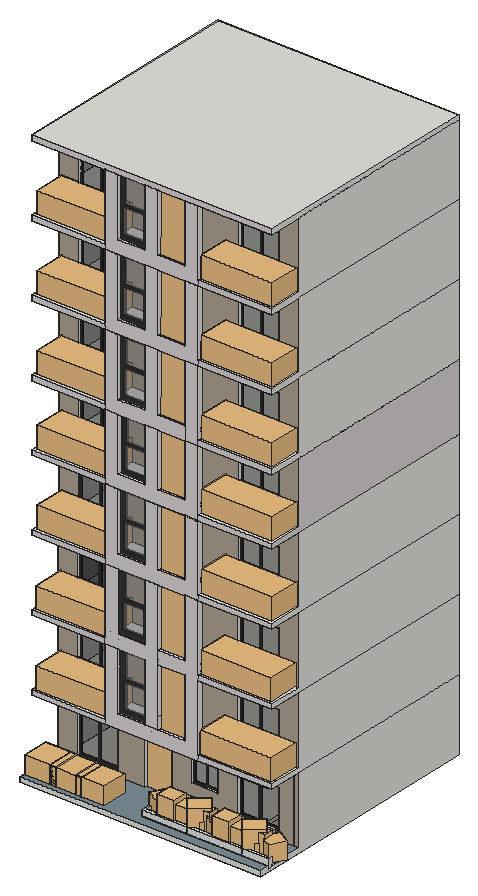
# SketchUp Ruby script. Lengths in inches.
U = 1.inch
M = Sketchup.active_model
def pt(a) = Geom::Point3d.new(a.map { |v| v * U })
def face(e, loops, mat)
  f = e.add_face(loops[0].map { |a| pt(a) })
  loops[1..].each { |l| e.add_face(l.map { |a| pt(a) }).erase! }
  f.material = f.back_material = mat if mat
  f
end
# faces: each face lists its corners as indices into pts; further lists are holes
def faces(e, pts, list, mat = nil) = list.each { |f| face(e, (f[0].is_a?(Array) ? f : [f]).map { |l| l.map { |i| pts[i] } }, mat) }
# xy, xz, yz: faces in a plane at the given z, y or x. An outline is a flat list of corners, or four numbers for a rectangle; further outlines are holes
def ring(l) = l.size == 4 ? [[l[0], l[1]], [l[2], l[1]], [l[2], l[3]], [l[0], l[3]]] : l.each_slice(2).to_a
def flat(e, list, mat, &to3) = list.each { |f| face(e, (f[0].is_a?(Array) ? f : [f]).map { |l| ring(l).map { |u, v| to3.(u, v) } }, mat) }
def xy(e, z, list, mat = nil) = flat(e, list, mat) { |x, y| [x, y, z] }
def xz(e, y, list, mat = nil) = flat(e, list, mat) { |x, z| [x, y, z] }
def yz(e, x, list, mat = nil) = flat(e, list, mat) { |y, z| [x, y, z] }
def lines(e, pts, list) = list.each { |a, b| e.add_line(pt(pts[a]), pt(pts[b])) }
# prism: a flat outline (further loops are holes) pulled along v
def prism(e, loops, v, mat = nil)
  f = face(e, loops, mat); d = Geom::Vector3d.new(v.map { |x| x * U })
  f.pushpull(f.normal.samedirection?(d) ? d.length : -d.length)
end
def box(e, o, s, mat = nil) = prism(e, [[o, [o[0] + s[0], o[1], o[2]], [o[0] + s[0], o[1] + s[1], o[2]], [o[0], o[1] + s[1], o[2]]]], [0, 0, s[2]], mat)
def at(x, y, z, deg = 0) = Geom::Transformation.translation(pt([x, y, z])) * Geom::Transformation.rotation(ORIGIN, Z_AXIS, deg.degrees)
def axes(o, x, y, z) = Geom::Transformation.new([*x, 0, *y, 0, *z, 0, *pt(o).to_a, 1])
def part(name) = M.definitions.add(name)
# library, detail: a bought-in or finely detailed component or shape, given as its bounding box
def library(name, o, s) = part(name).tap { |d| box(d.entities, o, s) }
def detail(e, o, s) = box(e.add_group.entities, o, s)
def put(e, d, t, mat = nil) = e.add_instance(d, t).tap { |i| i.material = mat if mat }
def group(e, t, mat = nil) = e.add_group.tap { |g| g.transformation = t; g.material = mat if mat }.entities
root = M.entities
M.materials.add("Glass_Tinted_Gray").color = [0, 0, 0]
M.materials["Glass_Tinted_Gray"].alpha = 0.125
M.materials.add("Material__1").color = [95, 70, 46]
M.materials.add("Windows").color = [58, 58, 58]
M.materials.add("[0035_Tan]").color = [174, 162, 146]
M.materials.add("[0135_DarkGray]").color = [81, 81, 81]
M.materials.add("[Blinds Cellular White]").color = [217, 211, 213]
M.materials.add("[Mirror 02]").color = [229, 229, 229]
M.materials.add("[Square Glass Tile 01]").color = [123, 142, 151]
M.materials.add("[Terrazzo Light Blue]").color = [196, 214, 227]
M.materials.add("[Translucent Glass Gray]").color = [128, 128, 128]
M.materials["[Translucent Glass Gray]"].alpha = 0.5
c1 = part("PENTEK_RP Fineline 50S_Sliding_DoorCase_E1")
box(c1.entities,[0,0,0],[1.51,3.66,99.27],"[0135_DarkGray]")
c2 = part("PENTEK_RP Fineline 50S_SlidingDooe_Case_E2")
box(c2.entities,[0,0,0],[96.25,3.66,1.51],"[0135_DarkGray]")
c3 = part("pentek_RP Fineline 50S_SlidingDoor_Case")
put(c3.entities,c1,at(97.76,0,0))
put(c3.entities,c2,at(1.51,0,0))
put(c3.entities,c1,at(0,0,0))
put(c3.entities,c2,at(1.51,0,97.76))
c4 = part("PENTEK_RP Fineline 50S_SlidingDoor_GlazingBead_2")
box(c4.entities,[0,0,0],[0.56,0.59,94.39],"[0135_DarkGray]")
c5 = part("PENTEK_RP Fineline 50S_SlidingDoor_Glass")
box(c5.entities,[0,0,0],[46.58,0.16,94.39],"Glass_Tinted_Gray")
c6 = part("PENTEK_RP Fineline 50S_SlidingDoor_GlazingBead")
box(c6.entities,[0,0,0],[45.47,0.59,0.56],"[0135_DarkGray]")
c7 = part("PENTEK_RP Fineline 50S_SlidingDoor_Leaf_E1")
xy(c7.entities,0,[[0,0,0.93,1.97],[0.93,1.57,1.49,1.97]],"[0135_DarkGray]")
xy(c7.entities,96.25,[[0,0,0.93,0,0.93,1.57,1.49,1.57,1.49,1.97,0,1.97]],"[0135_DarkGray]")
xz(c7.entities,0,[[0,0,0.93,96.25]],"[0135_DarkGray]")
xz(c7.entities,1.57,[[0.93,0,1.49,95.32],[0.93,95.32,1.49,96.25]],"[0135_DarkGray]")
xz(c7.entities,1.97,[[0,0,1.49,96.25]],"[0135_DarkGray]")
yz(c7.entities,0,[[0,0,1.97,96.25]],"[0135_DarkGray]")
yz(c7.entities,0.93,[[0,0,1.57,0.93],[0,0.93,1.57,95.32],[0,95.32,1.57,96.25]],"[0135_DarkGray]")
yz(c7.entities,1.49,[[1.57,0,1.97,95.32],[1.57,95.32,1.97,96.25]],"[0135_DarkGray]")
c8 = part("PENTEK_RP Fineline 50S_SlidingDoor_Leaf_E2")
xy(c8.entities,0,[[0,0,0,1.57,0.56,1.57,0.56,1.97,46.02,1.97,46.02,1.57,46.58,1.57,46.58,0]],"[0135_DarkGray]")
xy(c8.entities,0.93,[[0,0,46.58,1.57]],"[0135_DarkGray]")
xy(c8.entities,1.49,[[0.56,1.57,46.02,1.97]],"[0135_DarkGray]")
xz(c8.entities,0,[[0,0,46.58,0.93]],"[0135_DarkGray]")
xz(c8.entities,1.57,[[0,0,0.56,0.93],[46.02,0,46.58,0.93],[0.56,0.93,46.02,1.49]],"[0135_DarkGray]")
xz(c8.entities,1.97,[[0.56,0,46.02,1.49]],"[0135_DarkGray]")
yz(c8.entities,0,[[0,0,1.57,0.93]],"[0135_DarkGray]")
yz(c8.entities,0.56,[[1.57,0,1.97,0.93],[1.57,0.93,1.97,1.49]],"[0135_DarkGray]")
yz(c8.entities,46.02,[[1.57,0,1.97,0.93],[1.57,0.93,1.97,1.49]],"[0135_DarkGray]")
yz(c8.entities,46.58,[[0,0,1.57,0.93]],"[0135_DarkGray]")
c9 = part("PENTEK_RP Fineline S_SlidingDoor_Leaf1")
put(c9.entities,c4,at(0.93,0,0.93))
put(c9.entities,c4,at(46.96,0,0.93))
put(c9.entities,c5,at(1.49,1.42,0.93))
put(c9.entities,c6,at(1.49,0,0.93))
put(c9.entities,c5,at(1.49,0.59,0.93),"[Terrazzo Light Blue]")
put(c9.entities,c7,at(0,0,0))
put(c9.entities,c7,axes([48.44,0,0],[-1,0,0],[0,1,0],[0,0,1]))
put(c9.entities,c8,axes([0.93,0,96.25],[1,0,0],[0,1,0],[0,0,-1]))
put(c9.entities,c8,at(0.93,0,0))
put(c9.entities,c6,at(1.49,0,94.77))
c10 = part("PENTEK_RP Fineline 50S_SlidingDoor_Leaf2")
put(c10.entities,c5,at(1.49,1.42,0.93))
put(c10.entities,c6,at(1.49,0,94.77))
put(c10.entities,c4,at(46.96,0,0.93))
put(c10.entities,c5,at(1.49,0.59,0.93),"[Mirror 02]")
put(c10.entities,c4,at(0.93,0,0.93))
put(c10.entities,c7,at(0,0,0))
put(c10.entities,c7,axes([48.44,0,0],[-1,0,0],[0,1,0],[0,0,1]))
put(c10.entities,c6,at(1.49,0,0.93))
put(c10.entities,c8,axes([0.93,0,96.25],[1,0,0],[0,1,0],[0,0,-1]))
put(c10.entities,c8,at(0.93,0,0))
c11 = part("PENTEK - Slimmest Steel Sliding Door / Window\#1")
put(c11.entities,c3,at(0,-1.88,-0.09))
put(c11.entities,c9,at(1.51,-2.27,1.42))
put(c11.entities,c10,at(49.32,-0.3,1.42))
c12 = library("PINTU 6 YA",[0,-0.6875,0],[35.83,8.07,80.71])
c13 = library("Double casement window",[0,0,0],[5.2,55.12,70.87])
c14 = part("Window 06")
g1 = group(c14.entities,at(-11,5.5,0,-90))
xy(g1,0,[[0,11,5.5,35]],"Windows")
xy(g1,2,[[0,13,5.5,33]],"Windows")
xy(g1,53,[[0,13,5.5,33]],"Windows")
xy(g1,55,[[0,11,5.5,35]],"Windows")
xz(g1,11,[[0,0,5.5,55]],"Windows")
xz(g1,13,[[0,2,5.5,53]],"Windows")
xz(g1,33,[[0,2,5.5,53]],"Windows")
xz(g1,35,[[0,0,5.5,55]],"Windows")
yz(g1,0,[[[11,0,35,55],[13,2,33,53]]],"Windows")
yz(g1,5.5,[[[11,0,35,55],[13,2,33,53]]],"Windows")
g2 = group(g1,at(2.75,2,2))
xy(g2,0,[[0,11,2,31]],"Windows")
xy(g2,1,[[0,12,1,30],[1,12,2,30]],"Windows")
xy(g2,25,[[0,12,1,30],[1,12,2,30]],"Windows")
xy(g2,26,[[0,11,2,31]],"Windows")
xz(g2,11,[[0,0,2,26]],"Windows")
xz(g2,12,[[0,1,1,25],[1,1,2,25]],"Windows")
xz(g2,30,[[0,1,1,25],[1,1,2,25]],"Windows")
xz(g2,31,[[0,0,2,26]],"Windows")
yz(g2,0,[[[11,0,31,26],[12,1,30,25]]],"Windows")
yz(g2,1,[[12,1,30,25]],"[Translucent Glass Gray]")
yz(g2,2,[[[11,0,31,26],[12,1,30,25]]],"Windows")
g3 = group(g1,at(0.75,2,27))
xy(g3,0,[[0,11,2,31]],"Windows")
xy(g3,1,[[0,12,1,30],[1,12,2,30]],"Windows")
xy(g3,25,[[0,12,1,30],[1,12,2,30]],"Windows")
xy(g3,26,[[0,11,2,31]],"Windows")
xz(g3,11,[[0,0,2,26]],"Windows")
xz(g3,12,[[0,1,1,25],[1,1,2,25]],"Windows")
xz(g3,30,[[0,1,1,25],[1,1,2,25]],"Windows")
xz(g3,31,[[0,0,2,26]],"Windows")
yz(g3,0,[[[11,0,31,26],[12,1,30,25]]],"Windows")
yz(g3,1,[[12,1,30,25]],"[Translucent Glass Gray]")
yz(g3,2,[[[11,0,31,26],[12,1,30,25]]],"Windows")
c15 = library("Areca palm plant",[0,0,0],[49.1,36.6,54.46])
c16 = library("Group20\#1",[-20.81,-17.08,3.79],[39.86,39.43,37.51])
c17 = library("Group\#130",[-7.34,-1.2,0],[38.67,35.81,49.04])
c18 = library("Group\#10",[-84.69,-90.07,-0.36],[176.51,175.13,171.4])
c19 = library("Group38\#2",[14.01,28.44,-23.43],[18.58,18.32,38.89])
c20 = library("Group\#8",[-84.69,-90.07,-0.36],[176.51,175.13,171.4])
c21 = library("Group\#9",[-7.34,-1.2,0],[38.67,35.81,49.04])
c22 = library("Group\#74",[-84.69,-90.07,-0.36],[176.51,175.13,171.4])
c23 = library("Group\#13",[0,0,0],[56.8,25.91,35.15])
c24 = library("Group\#25",[0,0,0],[127.5,55.73,38.5])
c25 = library("Group\#23",[0,0,0],[127.5,55.73,38.5])
c26 = library("Group\#28",[0,0,0],[127.5,55.55,38.5])
c27 = library("Group\#24",[0,0,0],[127.5,55.55,38.5])
xy(root,-9,[[0,0,432,445.5]])
xy(root,-4,[[4.92,17.8,139.86,50.93],[204,17.8,432,50.93]])
xy(root,0,[[0,85.5,0,445.5,423,445.5,423,436.5,9,436.5,9,85.5],[9,85.5,156,94.5],[204,85.5,351,94.5],[351,85.5,360,94.5],[360,85.5,423,94.5],
  [351,94.5,360,436.5],[360,94.5,423,436.5]])
xy(root,0,[[[0,0,432,0,432,17.8,204,17.8,204,50.93,432,50.93,432,85.5,204,85.5,204,94.5,156,94.5,156,85.5,0,85.5],[4.92,17.8,139.86,50.93]]],"[Square Glass Tile 01]")
xy(root,9.75,[[36,85.5,108,94.5]])
xy(root,13.24,[[324,85.5,396,94.5]])
xy(root,36,[[240,85.5,288,94.5]])
xy(root,81.75,[[36,85.5,108,94.5]])
xy(root,84,[[156,85.5,204,94.5],[240,85.5,288,94.5]])
xy(root,85.24,[[324,85.5,396,94.5]])
xy(root,120,[[0,25.5,423,85.5],[423,25.5,432,85.5],[0,85.5,0,445.5,423,445.5,423,436.5,9,436.5,9,94.5,423,94.5,423,85.5],[423,85.5,432,445.5],[9,94.5,423,436.5]])
xy(root,129,[[0,25.5,132,34.5],[300,25.5,432,34.5],[0,34.5,9,85.5],[9,34.5,423,85.5],[423,34.5,432,85.5],
  [156,85.5,204,94.5],[9,94.5,423,436.5]])
xy(root,138,[[36,85.5,108,94.5],[324,85.5,396,94.5]])
xy(root,144,[[156,25.5,204,34.5],[228,25.5,276,34.5]])
xy(root,210,[[36,85.5,108,94.5],[156,85.5,204,94.5],[324,85.5,396,94.5]])
xy(root,249,[[0,25.5,0,85.5,300,85.5,300,34.5,276,34.5,276,25.5,228,25.5,228,34.5,132,34.5,132,25.5],[132,25.5,156,34.5],[156,25.5,204,34.5],[300,25.5,432,85.5],[[0,85.5,432,445.5],[9,94.5,423,436.5]]])
xy(root,258,[[0,25.5,132,25.5,132,34.5,9,34.5,9,85.5,0,85.5],[300,25.5,432,25.5,432,85.5,423,85.5,423,34.5,300,34.5],[9,34.5,423,85.5],[9,94.5,423,436.5]])
xy(root,270,[[36,85.5,108,94.5],[324,85.5,396,94.5]])
xy(root,273,[[228,25.5,276,34.5]])
xy(root,342,[[36,85.5,108,94.5],[324,85.5,396,94.5]])
xy(root,378,[[0,25.5,0,85.5,432,85.5,432,25.5,300,25.5,300,34.5,132,34.5,132,25.5],[141.5,25.5,156,34.5],[156,25.5,204,34.5],[204,25.5,228,34.5],[228,25.5,276,34.5],
  [276,25.5,300,34.5],[[0,85.5,432,445.5],[9,94.5,423,436.5]]])
xy(root,387,[[0,25.5,132,25.5,132,34.5,9,34.5,9,86.9375,0,86.9375],[300,25.5,432,25.5,432,86.9375,423,86.9375,423,34.5,300,34.5],[9,34.5,423,34.5,423,86.9375,204,86.9375,204,94.5,156,94.5,156,86.9375,9,86.9375],[9,94.5,423,436.5]])
xy(root,399,[[36,86.9375,108,94.5],[324,86.9375,396,94.5]])
xy(root,402,[[156,25.5,204,34.5],[228,25.5,276,34.5]])
xy(root,471,[[36,86.9375,108,94.5],[156,86.9375,204,94.5],[324,86.9375,396,94.5]])
xy(root,507,[[0,25.5,9,86.9375],[9,25.5,9,86.9375,423,86.9375,423,25.5,276,25.5,276,34.5,228,34.5,228,25.5],[156,25.5,204,34.5],[228,25.5,276,34.5],[423,25.5,432,86.9375],
  [0,86.9375,9,86.9375,9,436.5,423,436.5,423,86.9375,432,86.9375,432,445.5,0,445.5],[9,86.9375,423,94.5],[9,94.5,423,436.5]])
xy(root,507.0625,[[132,25.5,300,34.5]])
xy(root,516,[[0,25.5,132,25.5,132,34.5,9,34.5,9,86.9375,0,86.9375],[300,25.5,432,25.5,432,86.9375,423,86.9375,423,34.5,300,34.5],[9,34.5,423,34.5,423,86.9375,204,86.9375,204,95.9375,156,95.9375,156,86.9375,9,86.9375],[9,95.9375,423,436.5]])
xy(root,528,[[36,86.9375,108,95.9375],[324,86.9375,396,95.9375]])
xy(root,531,[[156,25.5,204,34.5],[228,25.5,276,34.5]])
xy(root,600,[[36,86.9375,108,95.9375],[156,86.9375,204,95.9375],[324,86.9375,396,95.9375]])
xy(root,627,[[0,25.5,9,86.9375],[9,25.5,9,86.9375,423,86.9375,423,25.5,300,25.5,300,34.5,132,34.5,132,25.5],[156,25.5,204,34.5],[228,25.5,276,34.5],[423,25.5,432,86.9375],
  [0,86.9375,9,86.9375,9,436.5,423,436.5,423,86.9375,432,86.9375,432,445.5,0,445.5],[9,86.9375,423,95.9375],[9,95.9375,423,436.5]])
xy(root,636,[[0,25.5,132,25.5,132,34.5,9,34.5,9,86.9375,0,86.9375],[300,25.5,432,25.5,432,86.9375,423,86.9375,423,34.5,300,34.5],[9,34.5,423,34.5,423,86.9375,204,86.9375,204,95.9375,156,95.9375,156,86.9375,9,86.9375],[9,95.9375,423,436.5]])
xy(root,648,[[36,86.9375,108,95.9375],[324,86.9375,396,95.9375]])
xy(root,651,[[156,25.5,204,34.5],[228,25.5,276,34.5]])
xy(root,720,[[36,86.9375,108,95.9375],[156,86.9375,204,95.9375],[324,86.9375,396,95.9375]])
xy(root,756,[[0,25.5,0,86.9375,432,86.9375,432,25.5,300,25.5,300,34.5,132,34.5,132,25.5],[132,25.5,156,34.5],[156,25.5,204,34.5],[204,25.5,228,34.5],[228,25.5,276,34.5],
  [[0,86.9375,432,445.5],[9,95.9375,423,436.5]]])
xy(root,765,[[0,25.5,132,25.5,132,34.5,9,34.5,9,86.9375,0,86.9375],[300,25.5,432,25.5,432,86.9375,423,86.9375,423,34.5,300,34.5],[9,34.5,423,34.5,423,86.9375,204,86.9375,204,95.9375,156,95.9375,156,86.9375,9,86.9375],[9,95.9375,423,436.5]])
xy(root,777,[[36,86.9375,108,95.9375],[324,86.9375,396,95.9375]])
xy(root,780,[[156,25.5,204,34.5],[228,25.5,276,34.5]])
xy(root,849,[[36,86.9375,108,95.9375],[156,86.9375,204,95.9375],[324,86.9375,396,95.9375]])
xy(root,885,[[0,25.5,0,86.9375,432,86.9375,432,25.5,300,25.5,300,34.5,132,34.5,132,25.5],[132,25.5,156,34.5],[156,25.5,204,34.5],[204,25.5,228,34.5],[228,25.5,276,34.5],
  [276,25.5,300,34.5],[[0,86.9375,432,445.5],[9,95.9375,423,436.5]]])
xy(root,894,[[0,25.5,132,25.5,132,34.5,9,34.5,9,86.9375,0,86.9375],[300,25.5,432,25.5,432,86.9375,423,86.9375,423,34.5,300,34.5],[9,34.5,423,34.5,423,86.9375,204,86.9375,204,95.9375,156,95.9375,156,86.9375,9,86.9375],[9,95.9375,423,436.5]])
xy(root,906,[[36,86.9375,108,95.9375],[324,86.9375,396,95.9375]])
xy(root,909,[[156,25.5,204.4375,34.5],[228,25.5,276,34.5]])
xy(root,919.875,[[9,95.9375,423,436.5]])
xy(root,978,[[36,86.9375,108,95.9375],[156,86.9375,204,95.9375],[324,86.9375,396,95.9375]])
xy(root,1014,[[0,25.5,0,86.9375,432,86.9375,432,25.5,300,25.5,300,34.5,132,34.5,132,25.5],[132,25.5,156,34.5],[156,25.5,204.4375,34.5],[204.4375,25.5,228,34.5],[228,25.5,276,34.5],
  [276,25.5,300,34.5],[[0,86.9375,432,445.5],[9,95.9375,423,436.5]]])
xy(root,1023,[[0,25.5,432,445.5]])
xz(root,0,[[0,-9,432,0]])
xz(root,17.8,[[4.92,-4,139.86,0],[204,-4,432,0]])
xz(root,25.5,[[132,507,300,507.0625]])
xz(root,25.5,[[0,120,132,129],[132,120,300,120,300,378,276,378,276,273,228,273,228,249,276,249,276,144,156,144,156,249,132,249],[300,120,432,129],[204,144,228,144,228,378,204,378,204,273,156,273,156,378,132,378,132,249,204,249],[0,249,132,258],
  [300,249,432,258],[0,378,132,387],[132,378,300,378,300,507,276,507,276,402,228,402,228,507,204,507,204,402,156,402,156,507,132,507],[300,378,432,387],[0,507,132,516],
  [300,507,432,516],[132,507.0625,300,507.0625,300,627,276,627,276,531,228,531,228,627,204,627,204,531,156,531,156,627,132,627],[0,627,276,627,276,651,228,651,228,756,204,756,204,651,156,651,156,756,132,756,132,636,0,636],[276,627,300,756],[300,627,432,636],
  [0,756,132,765],[132,756,300,756,300,885,276,885,276,780,228,780,228,885,204,885,204,780,156,780,156,885,132,885],[300,756,432,765],[0,885,132,894],[132,885,300,885,300,1014,276,1014,276,909,228,909,228,1014,204.4375,1014,204.4375,909,156,909,156,1014,132,1014],
  [300,885,432,894],[0,1014,432,1023]],"[Blinds Cellular White]")
xz(root,34.5,[[132,129,300,138],[132,138,132,165,156,165,156,144,204,144,204,165,228,165,228,144,276,144,276,165,300,165,300,138],[132,165,156,249],[204,165,228,249],[276,165,300,249],
  [132,258,141.5,378],[141.5,258,204,264.125],[204,258,204,264.125,156,264.125,156,273,204,273,204,378,228,378,228,258],[228,258,228,273,276,273,276,378,300,378,300,258],[141.5,264.125,156,273],
  [141.5,273,156,378],[[132,387,300,507.0625],[156,402,204,507],[228,402,276,507]],[132,516,132,627,156,627,156,531,204,531,204,627,228,627,228,531,276,531,276,627,300,627,300,516],[132,636,132,756,156,756,156,651,204,651,204,756,228,756,228,651,276,651,276,636],[276,636,300,756],
  [132,765,132,885,156,885,156,780,204,780,204,885,228,885,228,780,276,780,276,885,300,885,300,765],[132,894,132,1014,156,1014,156,909,204.4375,909,204.4375,1014,228,1014,228,909,276,909,276,1014,300,1014,300,894]])
xz(root,50.93,[[4.92,-4,139.86,0],[204,-4,432,0]])
xz(root,85.5,[[156,258,204,342]])
xz(root,85.5,[[[0,0,156,0,156,84,204,84,204,0,423,0,423,120,0,120],[36,9.75,108,81.75],[324,13.24,396,85.24],[240,36,288,84]],[423,0,432,120],[[0,129,156,129,156,210,204,210,204,129,432,129,432,249,0,249],[36,138,108,210],[324,138,396,210]],[[0,258,156,258,156,342,204,342,204,258,432,258,432,378,0,378],[36,270,108,342],[324,270,396,342]]],"[0035_Tan]")
xz(root,86.9375,[[[0,387,156,387,156,471,204,471,204,387,432,387,432,507,0,507],[36,399,108,471],[324,399,396,471]],[[0,516,156,516,156,600,204,600,204,516,432,516,432,627,0,627],[36,528,108,600],[324,528,396,600]],[[0,636,156,636,156,720,204,720,204,636,432,636,432,756,0,756],[36,648,108,720],[324,648,396,720]],[[0,765,156,765,156,849,204,849,204,765,432,765,432,885,0,885],[36,777,108,849],[324,777,396,849]],[[0,894,156,894,156,978,204,978,204,894,432,894,432,1014,0,1014],[36,906,108,978],[324,906,396,978]]],"[0035_Tan]")
xz(root,94.5,[[[9,0,9,120,423,120,423,0,204,0,204,84,156,84,156,0],[36,9.75,108,81.75],[324,13.24,396,85.24],[240,36,288,84]],[[9,129,9,249,423,249,423,129,204,129,204,210,156,210,156,129],[36,138,108,210],[324,138,396,210]],[[9,258,423,378],[36,270,108,342],[324,270,396,342]],[[9,387,9,507,423,507,423,387,204,387,204,471,156,471,156,387],[36,399,108,471],[324,399,396,471]]])
xz(root,95.9375,[[[9,516,9,627,423,627,423,516,204,516,204,600,156,600,156,516],[36,528,108,600],[324,528,396,600]],[[9,636,9,756,423,756,423,636,204,636,204,720,156,720,156,636],[36,648,108,720],[324,648,396,720]],[[9,765,9,885,423,885,423,765,204,765,204,849,156,849,156,765],[36,777,108,849],[324,777,396,849]],[9,894,9,919.875,36,919.875,36,906,108,906,108,919.875,156,919.875,156,894],[204,894,204,919.875,324,919.875,324,906,396,906,396,919.875,423,919.875,423,894],
  [9,919.875,9,1014,423,1014,423,919.875,396,919.875,396,978,324,978,324,919.875,204,919.875,204,978,156,978,156,919.875,108,919.875,108,978,36,978,36,919.875]])
xz(root,436.5,[[9,0,351,120],[351,0,423,120],[9,129,423,249],[9,258,423,378],[9,387,423,507],
  [9,516,423,627],[9,636,423,756],[9,765,423,885],[9,894,423,919.875],[9,919.875,423,1014]])
xz(root,445.5,[[0,-9,0,0,423,0,423,120,432,120,432,-9],[0,0,423,120],[0,120,432,249],[0,249,432,356.625],[0,356.625,432,378],
  [0,378,432,507],[0,507,432,627],[0,627,432,756],[0,756,432,885],[0,885,432,1014],
  [0,1014,432,1023]])
yz(root,0,[[0,-9,445.5,0],[85.5,0,445.5,120],[25.5,120,25.5,129,85.5,129,85.5,249,445.5,249,445.5,120],[25.5,249,85.5,258],[85.5,249,445.5,378],
  [25.5,378,85.5,387],[85.5,378,85.5,387,86.9375,387,86.9375,507,445.5,507,445.5,378],[86.9375,507,445.5,627],[25.5,627,86.9375,636],[86.9375,627,445.5,756],
  [25.5,756,86.9375,765],[86.9375,756,445.5,885],[25.5,885,86.9375,894],[86.9375,885,445.5,1014],[25.5,1014,445.5,1023]])
yz(root,0,[[25.5,507,86.9375,516]],"[Blinds Cellular White]")
yz(root,4.92,[[17.8,-4,50.93,0]])
yz(root,9,[[94.5,0,436.5,120],[94.5,129,436.5,249],[94.5,258,436.5,378],[94.5,387,436.5,507],[95.9375,516,436.5,627],
  [95.9375,636,436.5,756],[95.9375,765,436.5,885],[95.9375,894,436.5,919.875],[95.9375,919.875,436.5,1014]])
yz(root,36,[[85.5,9.75,94.5,81.75],[85.5,138,94.5,210],[85.5,270,94.5,342],[86.9375,399,94.5,471],[86.9375,528,95.9375,600],
  [86.9375,648,95.9375,720],[86.9375,777,95.9375,849],[86.9375,906,95.9375,978]])
yz(root,108,[[85.5,9.75,94.5,81.75],[85.5,138,94.5,210],[85.5,270,94.5,342],[86.9375,399,94.5,471],[86.9375,528,95.9375,600],
  [86.9375,648,95.9375,720],[86.9375,777,95.9375,849],[86.9375,906,95.9375,978]])
yz(root,132,[[25.5,129,34.5,138],[25.5,138,34.5,249],[25.5,258,34.5,378],[25.5,387,34.5,507.0625],[25.5,516,34.5,627],
  [25.5,636,34.5,756],[25.5,765,34.5,885],[25.5,894,34.5,1014]])
yz(root,139.86,[[17.8,-4,50.93,0]])
yz(root,156,[[85.5,0,94.5,84],[85.5,129,94.5,210],[25.5,144,34.5,249],[86.9375,387,94.5,471],[25.5,402,34.5,507],
  [86.9375,516,95.9375,600],[25.5,531,34.5,627],[86.9375,636,95.9375,720],[25.5,651,34.5,756],[86.9375,765,95.9375,849],
  [25.5,780,34.5,885],[86.9375,894,95.9375,978],[25.5,909,34.5,1014]])
yz(root,204,[[17.8,-4,50.93,0],[85.5,0,94.5,84],[85.5,129,94.5,210],[25.5,144,34.5,249],[25.5,273,34.5,378],
  [86.9375,387,94.5,471],[25.5,402,34.5,507],[86.9375,516,95.9375,600],[25.5,531,34.5,627],[86.9375,636,95.9375,720],
  [25.5,651,34.5,756],[86.9375,765,95.9375,849],[25.5,780,34.5,885],[86.9375,894,95.9375,978]])
yz(root,204.4375,[[25.5,909,34.5,1014]])
yz(root,228,[[25.5,144,34.5,165],[25.5,165,34.5,249],[25.5,273,34.5,378],[25.5,402,34.5,507],[25.5,531,34.5,627],
  [25.5,651,34.5,756],[25.5,780,34.5,885],[25.5,909,34.5,1014]])
yz(root,240,[[85.5,36,94.5,76.3125],[85.5,76.3125,94.5,84]])
yz(root,276,[[25.5,144,34.5,249],[25.5,273,34.5,378],[25.5,402,34.5,507],[25.5,531,34.5,627],[25.5,651,34.5,756],
  [25.5,780,34.5,885],[25.5,909,34.5,1014]])
yz(root,288,[[85.5,36,94.5,84]])
yz(root,300,[[25.5,129,34.5,249],[25.5,258,34.5,378],[25.5,387,34.5,507.0625],[25.5,516,34.5,627],[25.5,636,34.5,756],
  [25.5,765,34.5,885],[25.5,894,34.5,1014]])
yz(root,324,[[85.5,13.24,94.5,85.24],[85.5,138,94.5,210],[85.5,270,94.5,342],[86.9375,399,94.5,471],[86.9375,528,95.9375,600],
  [86.9375,648,95.9375,720],[86.9375,777,95.9375,849],[86.9375,906,95.9375,978]])
yz(root,396,[[85.5,13.24,94.5,85.24],[85.5,138,94.5,210],[85.5,270,94.5,342],[86.9375,399,94.5,471],[86.9375,528,95.9375,600],
  [86.9375,648,95.9375,720],[86.9375,777,95.9375,849],[86.9375,906,95.9375,978]])
yz(root,423,[[85.5,0,94.5,120],[94.5,0,436.5,120],[94.5,129,436.5,249],[94.5,258,436.5,378],[94.5,387,436.5,507],
  [95.9375,516,436.5,627],[95.9375,636,436.5,756],[95.9375,765,436.5,885],[95.9375,894,436.5,919.875],[95.9375,919.875,436.5,1014]])
yz(root,432,[[0,-9,445.5,-9,445.5,120,85.5,120,85.5,0,50.93,0,50.93,-4,17.8,-4,17.8,0,0,0],[25.5,120,445.5,120,445.5,249,85.5,249,85.5,129,25.5,129],[25.5,249,445.5,249,445.5,378,85.5,378,85.5,258,25.5,258],[25.5,378,445.5,378,445.5,507,86.9375,507,86.9375,387,25.5,387],[25.5,627,445.5,627,445.5,756,86.9375,756,86.9375,636,25.5,636],
  [25.5,756,445.5,756,445.5,885,86.9375,885,86.9375,765,25.5,765],[25.5,885,445.5,885,445.5,1014,86.9375,1014,86.9375,894,25.5,894],[25.5,1014,445.5,1023]])
yz(root,432,[[25.5,507,445.5,507,445.5,627,86.9375,627,86.9375,516,25.5,516]],"[Blinds Cellular White]")
p = [[316.24,-369.13,37.28],[315.96,-369.17,37.62],[216,34.5,138],[216,25.5,138],[1173.34,27.58,14.7],[1173.34,27.58,9.22],
  [1148.99,27.58,9.22],[1148.99,27.58,14.7],[1146.45,26.4,101.9375],[1146.45,27.58,101.9375],[1175.7,26.4,101.9375],[1175.7,27.58,101.9375],
  [141.5,25.5,273],[141.5,34.5,273],[156,25.5,264.125],[156,34.5,264.125],[132,25.5,627.9],[132,25.5,636]]
lines(root,p,[[0,1],[2,3],[4,5],[5,6],[6,7],[8,9],[10,11],[12,13],[14,15],[16,17]])
put(root,c11,axes([36,89.95,9.82],[0.72528,0,0],[0,0.64566,0],[0,0,0.72528]))
put(root,c11,axes([322.91,91.47,12.21],[0.72528,0,0],[0,0.64566,0],[0,0,0.72528]))
put(root,c11,axes([240,90.97,36.04],[0.48129,0,0],[0,0.42846,0],[0,0,0.48129]))
put(root,c12,axes([156,90,0],[1.33967,0,0],[0,1,0],[0,0,1.03]))
put(root,c11,axes([322.91,92.3,140.46],[0.72528,0,0],[0,0.64566,0],[0,0,0.72528]))
put(root,c11,axes([36,90.78,138.07],[0.72528,0,0],[0,0.64566,0],[0,0,0.72528]))
put(root,c13,axes([227.02,30.8,246.54],[0.01234,0.72173,-0.00323],[0.87571,-0.01494,0.00812],[0.01332,-0.00671,-1.44857]))
put(root,c14,axes([156,30,144],[2.0724,0,0],[0,1.57,0],[0,0,1.90909]))
put(root,c12,axes([156,90,129],[1.33967,0,0],[0,1,0],[0,0,1.03]))
put(root,c11,axes([36,91.42,270.07],[0.72528,0,0],[0,0.64566,0],[0,0,0.72528]))
put(root,c11,axes([324,91.47,270.07],[0.72528,0,0],[0,0.64566,0],[0,0,0.72528]))
put(root,c14,axes([154.26,30,273],[2.0724,0,0],[0,1.57,0],[0,0,1.90909]))
put(root,c13,axes([227.02,30.8,375.52],[0.01234,0.72173,-0.00323],[0.87571,-0.01494,0.00812],[0.01332,-0.00671,-1.44857]))
put(root,c11,axes([36,90.29,270.07],[0.72528,0,0],[0,0.64566,0],[0,0,0.72528]))
put(root,c11,axes([36,91.21,399.07],[0.72528,0,0],[0,0.64566,0],[0,0,0.72528]))
put(root,c11,axes([324,91.21,399.07],[0.72528,0,0],[0,0.64566,0],[0,0,0.72528]))
put(root,c12,axes([156,90,133.5625],[1.33967,0,0],[0,1,0],[0,0,1.03]))
put(root,c12,axes([156,90,387],[1.33967,0,0],[0,1,0],[0,0,1.03]))
put(root,c14,axes([156,30,402],[2.0724,0,0],[0,1.57,0],[0,0,1.90909]))
put(root,c13,axes([227.02,30.8,504.6],[0.01234,0.72173,-0.00323],[0.87571,-0.01494,0.00812],[0.01332,-0.00671,-1.44857]))
put(root,c11,axes([36,92.9,528.07],[0.72528,0,0],[0,0.64566,0],[0,0,0.72528]))
put(root,c11,axes([324,92.65,528.07],[0.72528,0,0],[0,0.64566,0],[0,0,0.72528]))
put(root,c12,axes([156,91.4375,516],[1.33967,0,0],[0,1,0],[0,0,1.03]))
put(root,c14,axes([157.15,31.04,531],[2.02432,0,0],[0,1.3816,0],[0,0,1.7472]))
put(root,c13,axes([227.02,30.8,633.6],[0.01234,0.72173,-0.00323],[0.87571,-0.01494,0.00812],[0.01332,-0.00671,-1.44857]))
put(root,c11,axes([36,92.9,648.07],[0.72528,0,0],[0,0.64566,0],[0,0,0.72528]))
put(root,c11,axes([324,92.9,648.07],[0.72528,0,0],[0,0.64566,0],[0,0,0.72528]))
put(root,c12,axes([156,91.4375,636],[1.33967,0,0],[0,1,0],[0,0,1.03]))
put(root,c12,axes([156,92.125,765],[1.33967,0,0],[0,1,0],[0,0,1.03]))
put(root,c11,axes([36,92.9,777.07],[0.72528,0,0],[0,0.64566,0],[0,0,0.72528]))
put(root,c11,axes([324,92.65,777.07],[0.72528,0,0],[0,0.64566,0],[0,0,0.72528]))
put(root,c12,axes([156,92.125,894],[1.33967,0,0],[0,1,0],[0,0,1.03]))
put(root,c11,axes([36,92.9,906.07],[0.72528,0,0],[0,0.64566,0],[0,0,0.72528]))
put(root,c11,axes([324,92.65,906.07],[0.72528,0,0],[0,0.64566,0],[0,0,0.72528]))
put(root,c14,axes([155.79,30,651],[2.0724,0,0],[0,1.57,0],[0,0,1.90909]))
put(root,c14,axes([154.26,30,780],[2.0724,0,0],[0,1.57,0],[0,0,1.90909]))
put(root,c14,axes([154.26,30,909],[2.0724,0,0],[0,1.57,0],[0,0,1.90909]))
put(root,c13,axes([227.02,30.48,753.52],[0.01234,0.72173,-0.00323],[0.87571,-0.01494,0.00812],[0.01332,-0.00671,-1.44857]))
put(root,c13,axes([227.06,30.48,882.65],[0.01234,0.72173,-0.00323],[0.87571,-0.01494,0.00812],[0.01332,-0.00671,-1.44857]))
put(root,c13,axes([227.02,30.48,1011.52],[0.01234,0.72173,-0.00323],[0.87571,-0.01494,0.00812],[0.01332,-0.00671,-1.44857]))
g4 = group(root,at(211.29,24,-4))
put(g4,c15,axes([74.23,-6.2,6.08],[0.54604,0.45017,0],[-0.51489,0.66137,0],[0,0,0.72]))
put(g4,c15,axes([173.17,-6.2,6.08],[0.54604,0.45017,0],[-0.51489,0.66137,0],[0,0,0.72]))
put(g4,c16,axes([150.45,18.97,4.77],[-0.826,0,0],[0,-0.85,0],[0,0,0.85]))
put(g4,c17,axes([140.8,24.9375,8],[-0.76769,0,0],[0,-0.79,0],[0,0,0.79]))
put(g4,c18,axes([158.88,14.93,6.05],[0.0835,-0.04961,0],[0.04821,0.08593,0],[0,0,0.10522]))
put(g4,c19,axes([229.29,-4.1,28.17],[0,0.8848,0],[-0.92,0,0],[0,0,0.85826]))
put(g4,c18,axes([110.36,17.19,6.07],[0.13689,-0.08133,0],[0.07903,0.14087,0],[0,0,0.1725]))
put(g4,c18,axes([212.82,17.19,6.07],[0.13689,-0.08133,0],[0.07903,0.14087,0],[0,0,0.1725]))
put(g4,c20,axes([185.36,14.93,6.05],[0.0835,-0.04961,0],[0.04821,0.08593,0],[0,0,0.10522]))
put(g4,c18,axes([11.42,17.19,6.07],[0.13689,-0.08133,0],[0.07903,0.14087,0],[0,0,0.1725]))
put(g4,c21,axes([41.86,24.9375,8],[-0.76769,0,0],[0,-0.79,0],[0,0,0.79]))
put(g4,c16,axes([51.52,18.97,4.77],[-0.826,0,0],[0,-0.85,0],[0,0,0.85]))
put(g4,c18,axes([139.38,14.93,6.05],[0.0835,-0.04961,0],[0.04821,0.08593,0],[0,0,0.10522]))
put(g4,c19,axes([130.35,-4.1,28.17],[0,0.8848,0],[-0.92,0,0],[0,0,0.85826]))
put(g4,c18,axes([40.45,14.93,6.05],[0.0835,-0.04961,0],[0.04821,0.08593,0],[0,0,0.10522]))
g5 = group(g4,at(220.88,-6.2,0))
xy(g5,0,[[-228.17,0,0,6],[-228.17,30,0,36]])
xy(g5,3,[[-228.17,6,0,30]])
xy(g5,7,[[-223.3125,6,-4.86,30]],"Material__1")
xy(g5,15,[[[-228.17,0,0,36],[-223.3125,6,-4.86,30]]])
xz(g5,0,[[-228.17,0,0,15]])
xz(g5,6,[[-228.17,0,0,3],[-223.3125,7,-4.86,15]])
xz(g5,30,[[-228.17,0,0,3],[-223.3125,7,-4.86,15]])
xz(g5,36,[[-228.17,0,0,15]])
yz(g5,-228.17,[[0,0,0,15,36,15,36,0,30,0,30,3,6,3,6,0]])
yz(g5,-223.3125,[[6,7,30,15]])
yz(g5,-4.86,[[6,7,30,15]])
yz(g5,0,[[0,0,6,0,6,3,30,3,30,0,36,0,36,15,0,15]])
put(g4,c18,axes([59.94,14.93,6.05],[0.0835,-0.04961,0],[0.04821,0.08593,0],[0,0,0.10522]))
put(g4,c22,axes([86.42,14.93,6.05],[0.0835,-0.04961,0],[0.04821,0.08593,0],[0,0,0.10522]))
put(root,c23,axes([0.01,9.43,-4],[1,0,0],[0,1.82,0],[0,0,1]))
put(root,c23,axes([45.58,9.43,-4.71],[1,0,0],[0,1.82,0],[0,0,1]))
put(root,c23,axes([92.01,9.43,-4.71],[0.89,0,0],[0,1.82,0],[0,0,1]))
put(root,c24,at(4.5,30,129))
put(root,c25,at(4.5,30,258))
put(root,c26,at(300,30,129))
put(root,c26,at(300,30.18,258))
put(root,c27,at(300,31.62,387))
put(root,c25,at(4.5,31.2,387))
put(root,c25,at(4.5,31.4375,516))
put(root,c27,at(300,31.62,516))
put(root,c25,at(4.5,31.4375,636))
put(root,c25,at(4.5,31.4375,765))
put(root,c25,at(4.5,31.2,894))
put(root,c27,at(300,31.62,636))
put(root,c27,at(300,31.39,765))
put(root,c27,at(300,31.39,894))
